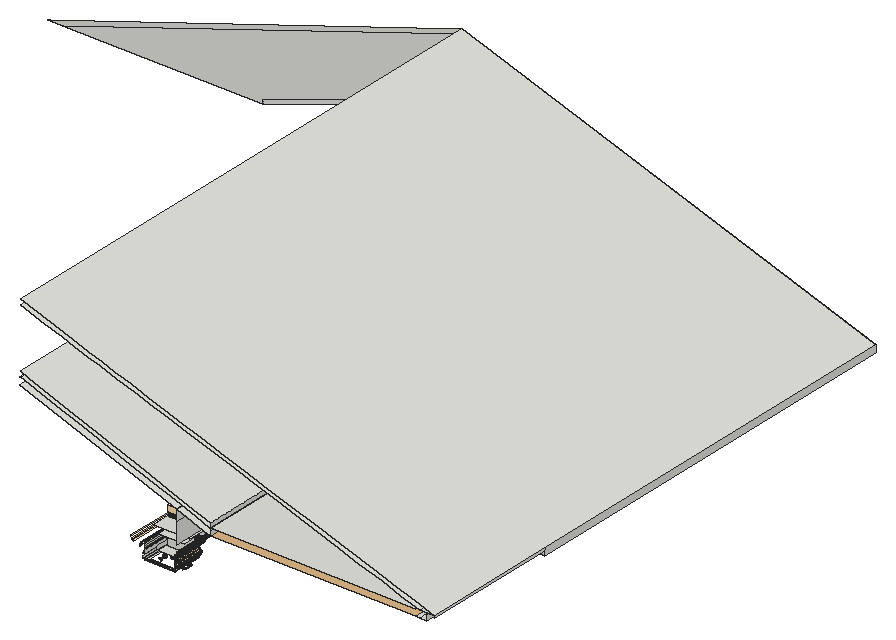
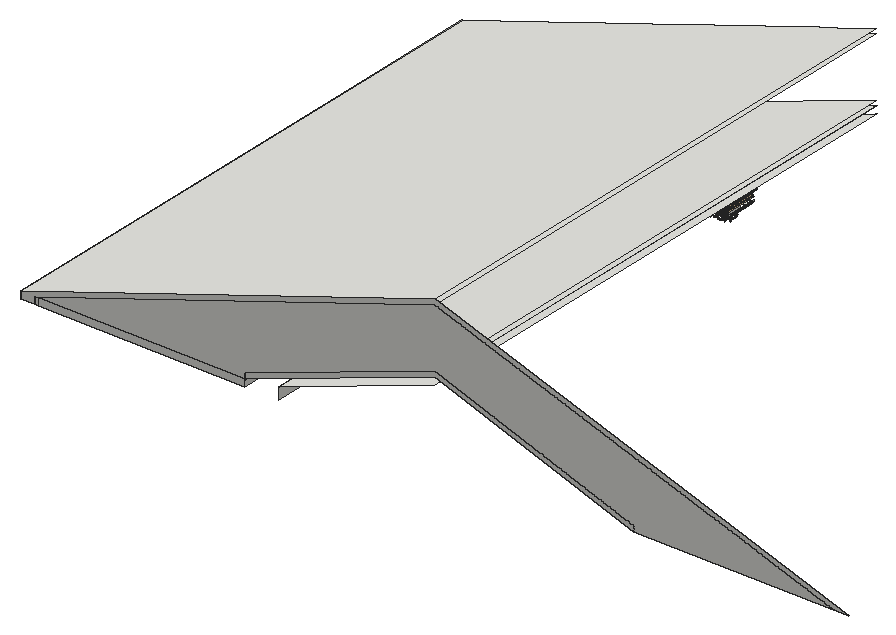
# SketchUp Ruby script. Lengths in inches.
U = 1.inch
M = Sketchup.active_model
def pt(a) = Geom::Point3d.new(a.map { |v| v * U })
def face(e, loops, mat)
  f = e.add_face(loops[0].map { |a| pt(a) })
  loops[1..].each { |l| e.add_face(l.map { |a| pt(a) }).erase! }
  f.material = f.back_material = mat if mat
  f
end
# faces: each face lists its corners as indices into pts; further lists are holes
def faces(e, pts, list, mat = nil) = list.each { |f| face(e, (f[0].is_a?(Array) ? f : [f]).map { |l| l.map { |i| pts[i] } }, mat) }
# xy, xz, yz: faces in a plane at the given z, y or x. An outline is a flat list of corners, or four numbers for a rectangle; further outlines are holes
def ring(l) = l.size == 4 ? [[l[0], l[1]], [l[2], l[1]], [l[2], l[3]], [l[0], l[3]]] : l.each_slice(2).to_a
def flat(e, list, mat, &to3) = list.each { |f| face(e, (f[0].is_a?(Array) ? f : [f]).map { |l| ring(l).map { |u, v| to3.(u, v) } }, mat) }
def xy(e, z, list, mat = nil) = flat(e, list, mat) { |x, y| [x, y, z] }
def xz(e, y, list, mat = nil) = flat(e, list, mat) { |x, z| [x, y, z] }
def yz(e, x, list, mat = nil) = flat(e, list, mat) { |y, z| [x, y, z] }
def lines(e, pts, list) = list.each { |a, b| e.add_line(pt(pts[a]), pt(pts[b])) }
# prism: a flat outline (further loops are holes) pulled along v
def prism(e, loops, v, mat = nil)
  f = face(e, loops, mat); d = Geom::Vector3d.new(v.map { |x| x * U })
  f.pushpull(f.normal.samedirection?(d) ? d.length : -d.length)
end
def box(e, o, s, mat = nil) = prism(e, [[o, [o[0] + s[0], o[1], o[2]], [o[0] + s[0], o[1] + s[1], o[2]], [o[0], o[1] + s[1], o[2]]]], [0, 0, s[2]], mat)
def at(x, y, z, deg = 0) = Geom::Transformation.translation(pt([x, y, z])) * Geom::Transformation.rotation(ORIGIN, Z_AXIS, deg.degrees)
def axes(o, x, y, z) = Geom::Transformation.new([*x, 0, *y, 0, *z, 0, *pt(o).to_a, 1])
def part(name) = M.definitions.add(name)
# library, detail: a bought-in or finely detailed component or shape, given as its bounding box
def library(name, o, s) = part(name).tap { |d| box(d.entities, o, s) }
def detail(e, o, s) = box(e.add_group.entities, o, s)
def put(e, d, t, mat = nil) = e.add_instance(d, t).tap { |i| i.material = mat if mat }
def group(e, t, mat = nil) = e.add_group.tap { |g| g.transformation = t; g.material = mat if mat }.entities
root = M.entities
M.materials.add("[0033_NavajoWhite]").color = [255, 222, 173]
M.materials.add("[0036_BurlyWood]").color = [222, 184, 135]
xy(root,94.95,[[[231.46,8.1,244.45,21.09],[232.25,9.67,243.67,19.51]]])
xy(root,95.99,[[231.46,14.59,244.45,21.09]])
xy(root,95.99,[[[230.94,7.58,244.97,21.61],[231.11,7.74,244.81,21.44]]],"[0033_NavajoWhite]")
xy(root,102.72,[[230.28,22.27,230.08,22.47,245.83,22.47,245.64,22.27]])
xy(root,102.72,[[230.08,22.47,229.3,23.25,246.62,23.25,245.83,22.47]],"[0033_NavajoWhite]")
xy(root,102.86,[[232.25,14.59,243.67,19.51]])
xy(root,105.42,[[230.08,14.59,245.83,22.47]])
xy(root,117,[[351.91,4.75,353.68,64.75],[353.68,4.75,356.68,64.75]])
xy(root,117,[[261.99,4.75,262.6,64.75],[262.6,4.75,351.91,64.75]],"[0036_BurlyWood]")
xy(root,120,[[262.52,4.75,262.6,244.75],[262.6,4.75,351.91,244.75],[353.68,4.75,360,64.75]])
xz(root,19.51,[[232.25,94.95,243.67,102.86]])
xz(root,21.09,[[231.46,94.95,244.45,95.1],[231.46,95.1,244.45,95.99],[231.46,95.99,244.45,97.5625],[231.46,97.5625,244.45,99.87],[231.46,99.87,244.45,100.56],
  [231.46,100.56,244.45,101.46]])
xz(root,21.61,[[230.94,95.99,244.97,96.66]])
xz(root,22.47,[[230.08,102.72,245.83,105.42]])
xz(root,24.44,[[228.12,105.42,247.8,108.125]],"[0033_NavajoWhite]")
xz(root,64.75,[[247.8,117,261.99,117,247.8,122.125],[353.68,117,356.68,120],[356.68,117,360,120]])
xz(root,244.75,[[353.68,117,353.68,120,180,177.89,6.32,120,0,120,180,180,360,120,360,117],[351.91,117,351.91,120,262.6,120,262.6,122.1,180,151.93,93.16,122.1,93.16,120,6.32,120,180,177.89,353.68,120,353.68,117],[262.6,117,351.91,120],[93.16,120,93.16,122.1,180,151.93,262.6,122.1,262.6,120,262.52,120,180,149.8,179.96,149.82]])
yz(root,230.94,[[7.58,95.99,21.61,96.66]])
yz(root,231.46,[[8.1,94.95,21.09,95.1],[8.1,95.1,21.09,95.99],[14.59,95.99,21.09,97.5625],[8.1,97.5625,21.09,99.87],[8.1,99.87,21.09,100.56],
  [8.1,100.56,21.09,101.46]])
yz(root,244.45,[[8.1,94.95,21.09,95.1],[8.1,95.1,21.09,95.99],[14.59,95.99,21.09,97.5625],[8.1,97.5625,21.09,99.87],[8.1,99.87,21.09,100.56],
  [8.1,100.56,21.09,101.46]])
yz(root,244.97,[[7.58,95.99,21.61,96.66]])
yz(root,245.24,[[7.32,96.99,21.87,96.99,21.875,97.11,7.31,97.11],[7.31,97.11,21.875,97.11,21.87,97.23,7.32,97.23]],"[0033_NavajoWhite]")
yz(root,245.83,[[6.73,100.89,22.46,100.89,22.47,101.01,6.72,101.01],[6.72,101.01,22.47,101.01,22.46,101.125,6.73,101.125]],"[0033_NavajoWhite]")
yz(root,247.8,[[4.75,108.125,64.75,117],[4.75,117,64.75,122.125],[64.75,117,244.75,122.125]])
yz(root,262.6,[[4.75,117,244.75,119],[4.75,119,244.75,119.97],[4.75,119.97,244.75,120],[4.75,120,244.75,122.1]])
yz(root,353.68,[[64.75,117,244.75,120]])
yz(root,356.68,[[4.75,117,64.75,119]])
yz(root,360,[[64.75,117,244.75,120],[4.75,119,64.75,120]])
p = [[235.01,18.5625,92.48],[235.01,18.53,92.25],[234.75,18.5625,92.25],[234.76,18.6,92.48],[235.25,18.6,92.48],[235.26,18.5625,92.25],
  [237.96,18.5625,92.48],[237.96,18.53,92.25],[237.7,18.5625,92.25],[237.71,18.6,92.48],[238.2,18.6,92.48],[238.21,18.5625,92.25],
  [240.91,18.5625,92.48],[240.91,18.53,92.25],[240.66,18.5625,92.25],[240.67,18.6,92.48],[241.16,18.6,92.48],[241.17,18.5625,92.25],
  [234.51,18.66,92.25],[234.53,18.69,92.48],[235.48,18.69,92.48],[235.5,18.66,92.25],[237.47,18.66,92.25],[237.48,18.69,92.48],
  [238.43,18.69,92.48],[238.45,18.66,92.25],[240.42,18.66,92.25],[240.4375,18.69,92.48],[241.39,18.69,92.48],[241.4,18.66,92.25],
  [234.31,18.82,92.25],[234.33,18.84,92.48],[235.68,18.84,92.48],[235.7,18.82,92.25],[237.26,18.82,92.25],[237.29,18.84,92.48],
  [238.63,18.84,92.48],[238.65,18.82,92.25],[240.22,18.82,92.25],[240.24,18.84,92.48],[241.58,18.84,92.48],[241.61,18.82,92.25],
  [234.15,19.02,92.25],[234.18,19.04,92.48],[235.83,19.04,92.48],[235.86,19.02,92.25],[237.11,19.02,92.25],[237.14,19.04,92.48],
  [238.78,19.04,92.48],[238.8125,19.02,92.25],[240.06,19.02,92.25],[240.09,19.04,92.48],[241.73,19.04,92.48],[241.76,19.02,92.25],
  [234.05,19.26,92.25],[234.09,19.27,92.48],[235.92,19.27,92.48],[235.96,19.26,92.25],[237.01,19.26,92.25],[237.04,19.27,92.48],
  [238.875,19.27,92.48],[238.91,19.26,92.25],[239.96,19.26,92.25],[239.99,19.27,92.48],[241.83,19.27,92.48],[241.86,19.26,92.25],
  [234.02,19.51,92.25],[234.05,19.51,92.48],[235.96,19.51,92.48],[235.99,19.51,92.25],[236.97,19.51,92.25],[237.01,19.51,92.48],
  [238.91,19.51,92.48],[238.94,19.51,92.25],[239.93,19.51,92.25],[239.96,19.51,92.48],[241.86,19.51,92.48],[241.9,19.51,92.25],
  [233.17,14.84,92.74],[233.2,14.85,92.51],[233.23,14.59,92.51],[233.2,14.59,92.74],[242.72,14.85,92.51],[242.75,14.84,92.74],
  [242.72,14.59,92.74],[242.68,14.59,92.51],[233.07,15.07,92.74],[233.1,15.08,92.51],[242.81,15.08,92.51],[242.84,15.07,92.74],
  [232.92,15.26,92.74],[232.95,15.29,92.51],[242.97,15.29,92.51],[242.99,15.26,92.74],[232.73,15.42,92.74],[232.74,15.44,92.51],
  [243.17,15.44,92.51],[243.19,15.42,92.74],[232.5,15.51,92.74],[232.5,15.54,92.51],[243.41,15.54,92.51],[243.42,15.51,92.74],
  [232.25,15.54,92.74],[232.25,15.58,92.51],[243.67,15.54,92.74],[243.67,15.58,92.51],[232.25,16.59,92.74],[232.5,16.625,92.74],
  [232.5,16.59,92.51],[232.25,16.5625,92.51],[232.73,16.72,92.74],[232.74,16.69,92.51],[243.42,16.625,92.74],[243.41,16.59,92.51],
  [243.17,16.69,92.51],[243.19,16.72,92.74],[243.67,16.59,92.74],[243.67,16.5625,92.51],[232.92,16.875,92.74],[232.95,16.85,92.51],
  [242.97,16.85,92.51],[242.99,16.875,92.74],[233.07,17.07,92.74],[233.1,17.05,92.51],[242.81,17.05,92.51],[242.84,17.07,92.74],
  [233.17,17.3,92.74],[233.2,17.29,92.51],[242.72,17.29,92.51],[242.75,17.3,92.74],[233.2,17.55,92.74],[233.23,17.55,92.51],
  [242.68,17.55,92.51],[242.72,17.55,92.74],[233.17,17.79,92.74],[233.2,17.8,92.51],[242.72,17.8,92.51],[242.75,17.79,92.74],
  [233.07,18.02,92.74],[233.1,18.04,92.51],[242.81,18.04,92.51],[242.84,18.02,92.74],[232.92,18.22,92.74],[232.95,18.24,92.51],
  [242.97,18.24,92.51],[242.99,18.22,92.74],[232.73,18.37,92.74],[232.74,18.4,92.51],[243.17,18.4,92.51],[243.19,18.37,92.74],
  [232.5,18.46,92.74],[232.5,18.5,92.51],[243.41,18.5,92.51],[243.42,18.46,92.74],[232.25,18.53,92.51],[232.25,18.5,92.74],
  [243.67,18.53,92.51],[243.67,18.5,92.74],[234.78,18.69,92.7],[234.58,18.78,92.7],[235.01,18.66,92.7],[235.23,18.69,92.7],
  [235.43,18.78,92.7],[237.74,18.69,92.7],[237.53,18.78,92.7],[237.96,18.66,92.7],[238.18,18.69,92.7],[238.38,18.78,92.7],
  [240.69,18.69,92.7],[240.48,18.78,92.7],[240.91,18.66,92.7],[241.13,18.69,92.7],[241.34,18.78,92.7],[234.4,18.91,92.7],
  [235.61,18.91,92.7],[237.36,18.91,92.7],[238.5625,18.91,92.7],[240.31,18.91,92.7],[241.51,18.91,92.7],[234.27,19.09,92.7],
  [235.74,19.09,92.7],[237.22,19.09,92.7],[238.7,19.09,92.7],[240.17,19.09,92.7],[241.65,19.09,92.7],[234.18,19.29,92.7],
  [235.83,19.29,92.7],[237.14,19.29,92.7],[238.78,19.29,92.7],[240.09,19.29,92.7],[241.73,19.29,92.7],[234.15,19.51,92.7],
  [235.86,19.51,92.7],[237.11,19.51,92.7],[238.8125,19.51,92.7],[240.06,19.51,92.7],[241.76,19.51,92.7],[233.07,14.8125,92.96],
  [233.1,14.59,92.96],[242.84,14.8125,92.96],[242.81,14.59,92.96],[232.99,15.02,92.96],[242.93,15.02,92.96],[232.85,15.2,92.96],
  [243.0625,15.2,92.96],[232.68,15.33,92.96],[243.24,15.33,92.96],[232.47,15.42,92.96],[243.45,15.42,92.96],[232.25,15.44,92.96],
  [243.67,15.44,92.96],[232.25,16.69,92.96],[232.47,16.72,92.96],[232.68,16.81,92.96],[243.45,16.72,92.96],[243.24,16.81,92.96],
  [243.67,16.69,92.96],[232.85,16.94,92.96],[243.0625,16.94,92.96],[232.99,17.12,92.96],[242.93,17.12,92.96],[233.07,17.32,92.96],
  [242.84,17.32,92.96],[233.1,17.55,92.96],[242.81,17.55,92.96],[233.07,17.77,92.96],[242.84,17.77,92.96],[232.99,17.97,92.96],
  [242.93,17.97,92.96],[232.85,18.15,92.96],[243.0625,18.15,92.96],[232.68,18.28,92.96],[243.24,18.28,92.96],[232.47,18.37,92.96],
  [243.45,18.37,92.96],[232.25,18.4,92.96],[243.67,18.4,92.96],[234.83,18.84,92.89],[234.66,18.91,92.89],[235.01,18.82,92.89],
  [235.1875,18.84,92.89],[235.35,18.91,92.89],[237.78,18.84,92.89],[237.61,18.91,92.89],[237.96,18.82,92.89],[238.14,18.84,92.89],
  [238.31,18.91,92.89],[240.73,18.84,92.89],[240.5625,18.91,92.89],[240.91,18.82,92.89],[241.09,18.84,92.89],[241.26,18.91,92.89],
  [234.51,19.02,92.89],[235.5,19.02,92.89],[237.47,19.02,92.89],[238.45,19.02,92.89],[240.42,19.02,92.89],[241.4,19.02,92.89],
  [234.4,19.17,92.89],[235.61,19.17,92.89],[237.36,19.17,92.89],[238.5625,19.17,92.89],[240.31,19.17,92.89],[241.51,19.17,92.89],
  [234.33,19.33,92.89],[235.68,19.33,92.89],[237.29,19.33,92.89],[238.63,19.33,92.89],[240.24,19.33,92.89],[241.58,19.33,92.89],
  [234.31,19.51,92.89],[235.7,19.51,92.89],[237.26,19.51,92.89],[238.65,19.51,92.89],[240.22,19.51,92.89],[241.61,19.51,92.89],
  [234.88,19.04,93.03],[234.76,19.09,93.03],[235.01,19.02,93.03],[235.13,19.04,93.03],[235.25,19.09,93.03],[237.83,19.04,93.03],
  [237.71,19.09,93.03],[237.96,19.02,93.03],[238.09,19.04,93.03],[238.2,19.09,93.03],[240.78,19.04,93.03],[240.67,19.09,93.03],
  [240.91,19.02,93.03],[241.04,19.04,93.03],[241.16,19.09,93.03],[234.66,19.17,93.03],[235.35,19.17,93.03],[237.61,19.17,93.03],
  [238.31,19.17,93.03],[240.5625,19.17,93.03],[241.26,19.17,93.03],[234.58,19.27,93.03],[235.43,19.27,93.03],[237.53,19.27,93.03],
  [238.38,19.27,93.03],[240.48,19.27,93.03],[241.34,19.27,93.03],[234.53,19.39,93.03],[235.48,19.39,93.03],[237.48,19.39,93.03],
  [238.43,19.39,93.03],[240.4375,19.39,93.03],[241.39,19.39,93.03],[234.51,19.51,93.03],[235.5,19.51,93.03],[237.47,19.51,93.03],
  [238.45,19.51,93.03],[240.42,19.51,93.03],[241.4,19.51,93.03],[232.92,14.77,93.15],[232.95,14.59,93.15],[242.99,14.77,93.15],
  [242.97,14.59,93.15],[232.85,14.94,93.15],[243.0625,14.94,93.15],[232.74,15.08,93.15],[243.17,15.08,93.15],[232.6,15.2,93.15],
  [243.32,15.2,93.15],[232.43,15.26,93.15],[243.49,15.26,93.15],[232.25,15.29,93.15],[243.67,15.29,93.15],[232.25,16.85,93.15],
  [232.43,16.875,93.15],[232.6,16.94,93.15],[243.49,16.875,93.15],[243.32,16.94,93.15],[243.67,16.85,93.15],[232.74,17.05,93.15],
  [243.17,17.05,93.15],[232.85,17.2,93.15],[243.0625,17.2,93.15],[232.92,17.37,93.15],[242.99,17.37,93.15],[232.95,17.55,93.15],
  [242.97,17.55,93.15],[232.92,17.73,93.15],[242.99,17.73,93.15],[232.85,17.89,93.15],[243.0625,17.89,93.15],[232.74,18.04,93.15],
  [243.17,18.04,93.15],[232.6,18.15,93.15],[243.32,18.15,93.15],[232.43,18.22,93.15],[243.49,18.22,93.15],[232.25,18.24,93.15],
  [243.67,18.24,93.15],[234.94,19.27,93.12],[234.88,19.29,93.12],[235.01,19.26,93.12],[235.07,19.27,93.12],[235.13,19.29,93.12],
  [237.89,19.27,93.12],[237.83,19.29,93.12],[237.96,19.26,93.12],[238.02,19.27,93.12],[238.09,19.29,93.12],[240.85,19.27,93.12],
  [240.78,19.29,93.12],[240.91,19.26,93.12],[240.98,19.27,93.12],[241.04,19.29,93.12],[234.83,19.33,93.12],[235.1875,19.33,93.12],
  [237.78,19.33,93.12],[238.14,19.33,93.12],[240.73,19.33,93.12],[241.09,19.33,93.12],[234.78,19.39,93.12],[235.23,19.39,93.12],
  [237.74,19.39,93.12],[238.18,19.39,93.12],[240.69,19.39,93.12],[241.13,19.39,93.12],[234.76,19.45,93.12],[235.25,19.45,93.12],
  [237.71,19.45,93.12],[238.2,19.45,93.12],[240.67,19.45,93.12],[241.16,19.45,93.12],[234.75,19.51,93.12],[235.26,19.51,93.12],
  [237.7,19.51,93.12],[238.21,19.51,93.12],[240.66,19.51,93.12],[241.17,19.51,93.12],[232.73,14.72,93.29],[232.74,14.59,93.29],
  [243.19,14.72,93.29],[243.17,14.59,93.29],[232.68,14.84,93.29],[243.24,14.84,93.29],[232.6,14.94,93.29],[243.32,14.94,93.29],
  [232.5,15.02,93.29],[243.42,15.02,93.29],[232.38,15.07,93.29],[243.54,15.07,93.29],[232.25,15.08,93.29],[243.67,15.08,93.29],
  [232.25,17.05,93.29],[232.38,17.07,93.29],[243.54,17.07,93.29],[243.67,17.05,93.29],[232.5,17.12,93.29],[232.6,17.2,93.29],
  [243.42,17.12,93.29],[243.32,17.2,93.29],[232.68,17.3,93.29],[243.24,17.3,93.29],[232.73,17.42,93.29],[243.19,17.42,93.29],
  [232.74,17.55,93.29],[243.17,17.55,93.29],[232.73,17.67,93.29],[243.19,17.67,93.29],[232.68,17.79,93.29],[243.24,17.79,93.29],
  [232.6,17.89,93.29],[243.32,17.89,93.29],[232.5,17.97,93.29],[243.42,17.97,93.29],[232.38,18.02,93.29],[232.25,18.04,93.29],
  [243.54,18.02,93.29],[243.67,18.04,93.29],[235.01,19.51,93.15],[237.96,19.51,93.15],[240.91,19.51,93.15],[232.5,14.66,93.38],
  [232.5,14.59,93.38],[243.42,14.66,93.38],[243.41,14.59,93.38],[232.43,14.77,93.38],[232.47,14.72,93.38],[243.45,14.72,93.38],
  [243.49,14.77,93.38],[232.32,14.84,93.38],[232.25,14.85,93.38],[232.38,14.8125,93.38],[243.54,14.8125,93.38],[243.6,14.84,93.38],
  [243.67,14.85,93.38],[232.25,17.29,93.38],[232.32,17.3,93.38],[232.38,17.32,93.38],[232.43,17.37,93.38],[243.54,17.32,93.38],
  [243.49,17.37,93.38],[243.6,17.3,93.38],[243.67,17.29,93.38],[232.47,17.42,93.38],[243.45,17.42,93.38],[232.5,17.48,93.38],
  [243.42,17.48,93.38],[232.5,17.55,93.38],[243.41,17.55,93.38],[232.5,17.61,93.38],[243.42,17.61,93.38],[232.47,17.67,93.38],
  [243.45,17.67,93.38],[232.43,17.73,93.38],[232.38,17.77,93.38],[243.49,17.73,93.38],[243.54,17.77,93.38],[232.32,17.79,93.38],
  [232.25,17.8,93.38],[243.6,17.79,93.38],[243.67,17.8,93.38],[232.25,14.59,93.41],[243.67,14.59,93.41],[232.25,17.55,93.41],
  [243.67,17.55,93.41],[231.45,8.09,95.25],[231.45,21.1,95.25],[231.46,21.09,95.1],[231.46,8.1,95.1],[244.45,8.1,95.1],
  [244.45,21.09,95.1],[244.47,21.1,95.25],[244.47,8.09,95.25],[231.43,8.06,95.4],[231.43,21.12,95.4],[244.49,21.12,95.4],
  [244.49,8.06,95.4],[244.52,21.15,95.53],[231.4,21.15,95.53],[244.55,21.1875,95.66],[231.36,21.1875,95.66],[244.6,21.24,95.77],
  [231.32,21.24,95.77],[231.26,7.9,95.86],[231.26,21.29,95.86],[231.32,7.95,95.77],[244.6,7.95,95.77],[244.65,21.29,95.86],
  [244.65,7.9,95.86],[231.2,7.84,95.93],[231.2,21.35,95.93],[244.71,21.35,95.93],[244.71,7.84,95.93],[244.78,21.41,95.98],
  [231.14,21.41,95.98],[231.11,7.74,95.99],[231.11,21.44,95.99],[231.14,7.78,95.98],[244.78,7.78,95.98],[244.81,21.44,95.99],
  [244.81,7.74,95.99],[245.1,7.45,96.68],[245.1,21.73,96.68],[245.14,21.78,96.72],[245.14,7.41,96.72],[245.04,7.51,96.66],
  [245.04,21.68,96.66],[230.87,21.68,96.66],[230.82,21.73,96.68],[230.77,21.78,96.72],[245.18,21.82,96.79],[230.73,21.82,96.79],
  [245.22,21.85,96.89],[230.7,21.85,96.89],[245.22,7.34,96.89],[245.24,21.87,96.99],[245.24,7.32,96.99],[230.68,21.87,96.99],
  [245.24,21.875,97.11],[230.67,21.875,97.11],[245.24,21.87,97.23],[230.68,21.87,97.23],[245.24,7.32,97.23],[245.22,21.85,97.34],
  [245.22,7.34,97.34],[230.7,21.85,97.34],[245.18,21.82,97.43],[230.73,21.82,97.43],[245.14,21.78,97.5],[230.77,21.78,97.5],
  [245.14,7.41,97.5],[245.1,21.73,97.55],[245.1,7.45,97.55],[245.04,21.68,97.5625],[245.04,7.51,97.5625],[230.82,21.73,97.55],
  [230.87,21.68,97.5625],[244.95,21.58,97.74],[244.95,7.61,97.74],[230.97,21.58,97.74],[231.0625,7.7,97.93],[231.0625,21.49,97.93],
  [230.97,7.61,97.74],[244.85,21.49,97.93],[244.85,7.7,97.93],[244.77,21.4,98.14],[244.77,7.78,98.14],[231.15,21.4,98.14],
  [231.22,7.86,98.375],[231.22,21.33,98.375],[231.15,7.78,98.14],[244.69,21.33,98.375],[244.69,7.86,98.375],[231.29,7.92,98.62],
  [231.29,21.26,98.62],[244.625,21.26,98.62],[244.625,7.92,98.62],[231.35,7.98,98.875],[231.35,21.2,98.875],[244.57,21.2,98.875],
  [244.57,7.98,98.875],[231.39,8.03,99.14],[231.39,21.16,99.14],[244.52,21.16,99.14],[244.52,8.03,99.14],[231.43,8.0625,99.42],
  [231.43,21.12,99.42],[244.49,21.12,99.42],[244.49,8.0625,99.42],[244.46,21.1,99.7],[231.45,21.1,99.7],[231.46,8.1,99.87],
  [231.46,21.09,99.87],[231.45,8.09,99.7],[244.46,8.09,99.7],[244.45,21.09,99.87],[244.45,8.1,99.87],[230.14,6.78,100.6875],
  [230.14,22.41,100.6875],[230.18,22.37,100.62],[230.18,6.82,100.62],[230.23,22.32,100.57],[230.23,6.86,100.57],[245.6875,6.86,100.57],
  [245.6875,22.32,100.57],[245.73,22.37,100.62],[245.73,6.82,100.62],[245.77,22.41,100.6875],[245.77,6.78,100.6875],[245.64,6.92,100.56],
  [245.64,22.27,100.56],[230.28,22.27,100.56],[245.81,22.44,100.78],[245.81,6.74,100.78],[230.11,22.44,100.78],[245.83,22.46,100.89],
  [230.09,22.46,100.89],[245.83,22.47,101.01],[230.08,22.47,101.01],[245.83,22.46,101.125],[230.09,22.46,101.125],[245.81,22.44,101.23],
  [230.11,22.44,101.23],[245.81,6.74,101.23],[245.77,22.41,101.33],[245.77,6.78,101.33],[230.14,22.41,101.33],[230.18,6.82,101.4],
  [230.18,22.37,101.4],[230.14,6.78,101.33],[245.73,22.37,101.4],[245.73,6.82,101.4],[230.23,6.86,101.44],[230.23,22.32,101.44],
  [245.6875,22.32,101.44],[245.6875,6.86,101.44],[245.64,22.27,101.46],[245.64,6.92,101.46],[230.28,22.27,101.46],[245.53,22.17,101.6],
  [245.53,7.02,101.6],[245.58,6.97,101.52],[245.58,22.22,101.52],[230.34,22.22,101.52],[230.38,22.17,101.6],[245.49,22.13,101.7],
  [245.49,7.06,101.7],[230.42,22.13,101.7],[245.46,22.1,101.82],[245.46,7.09,101.82],[230.45,22.1,101.82],[230.45,7.09,101.82],
  [230.47,7.11,101.95],[230.47,22.08,101.95],[245.44,22.08,101.95],[245.44,7.11,101.95],[230.48,7.11,102.09],[230.48,22.07,102.09],
  [245.4375,22.07,102.09],[245.4375,7.11,102.09],[230.47,7.11,102.23],[230.47,22.08,102.23],[245.44,22.08,102.23],[245.44,7.11,102.23],
  [230.45,7.09,102.36],[230.45,22.1,102.36],[245.46,22.1,102.36],[245.46,7.09,102.36],[245.49,22.13,102.48],[245.49,7.06,102.48],
  [230.42,22.13,102.48],[245.53,22.17,102.58],[245.53,7.02,102.58],[230.38,22.17,102.58],[245.58,22.22,102.66],[245.58,6.97,102.66],
  [230.34,22.22,102.66],[246.78,5.77,102.7],[246.78,23.41,102.7],[246.94,23.58,102.73],[246.94,5.61,102.73],[246.62,5.93,102.72],
  [246.62,23.25,102.72],[230.28,22.27,102.72],[245.64,22.27,102.72],[229.3,23.25,102.72],[229.14,23.41,102.7],[228.98,23.58,102.73],
  [228.82,23.73,102.82],[247.1,23.73,102.82],[247.1,5.45,102.82],[247.25,23.88,102.96],[247.25,5.3,102.96],[228.67,23.88,102.96],
  [228.53,5.17,103.15],[228.53,24.02,103.15],[228.67,5.3,102.96],[247.38,24.02,103.15],[247.38,5.17,103.15],[247.51,24.14,103.39],
  [247.51,5.05,103.39],[228.41,24.14,103.39],[247.61,24.24,103.68],[247.61,4.94,103.68],[228.31,24.24,103.68],[228.22,4.86,103.99],
  [228.22,24.33,103.99],[228.31,4.94,103.68],[247.7,24.33,103.99],[247.7,4.86,103.99],[247.76,24.39,104.33],[247.76,4.79,104.33],
  [228.16,24.39,104.33],[247.8,24.43,104.6875],[247.8,4.75,104.6875],[228.12,24.43,104.6875],[228.11,4.74,105.05],[228.11,24.45,105.05],
  [228.12,4.75,104.6875],[247.8125,24.45,105.05],[247.8125,4.74,105.05],[247.8,24.44,105.42],[247.8,4.75,105.42],[228.12,24.44,105.42],
  [261.99,4.75,117],[247.8,4.75,122.125],[247.8,64.75,122.125],[261.99,64.75,117],[180,4.75,177.89],[190.82,4.75,174.29],
  [198.59,4.75,171.69],[203.74,4.75,169.98],[209.51,4.75,168.05],[214.75,4.75,166.31],[222.01,4.75,163.89],[229.64,4.75,161.35],
  [236.39,4.75,159.09],[244.33,4.75,156.45],[252.34,4.75,153.78],[262.54,4.75,150.38],[271.37,4.75,147.4375],[281.28,4.75,144.13],
  [291.76,4.75,140.64],[303.43,4.75,136.75],[316.44,4.75,132.41],[327.22,4.75,128.82],[337.3,4.75,125.46],[345.49,4.75,122.73],
  [353.68,4.75,120],[353.68,64.75,120],[353.68,244.75,120],[180,244.75,177.89],[351.8125,4.75,122.73],[360,4.75,120],
  [360,64.75,120],[360,244.75,120],[180,244.75,180],[180,4.75,180],[197,4.75,174.33],[204.77,4.75,171.74],
  [209.93,4.75,170.02],[215.69,4.75,168.1],[221.07,4.75,166.31],[228.33,4.75,163.89],[235.96,4.75,161.35],[242.72,4.75,159.09],
  [250.66,4.75,156.45],[258.67,4.75,153.78],[268.86,4.75,150.38],[277.69,4.75,147.4375],[287.61,4.75,144.13],[298.08,4.75,140.64],
  [309.76,4.75,136.75],[322.77,4.75,132.41],[333.54,4.75,128.82],[343.625,4.75,125.46],[180,244.75,149.8],[180,4.75,149.8],
  [186.55,4.75,147.4375],[195.7,4.75,144.13],[205.37,4.75,140.64],[216.15,4.75,136.75],[228.15,4.75,132.41],[238.1,4.75,128.82],
  [247.4,4.75,125.46],[256.71,4.75,122.1],[262.52,4.75,120],[262.52,244.75,120],[262.6,4.75,119.97],[262.6,244.75,119.97],
  [184.29,4.75,150.38],[180,4.75,151.93],[180,244.75,151.93],[262.6,244.75,122.1],[262.6,4.75,122.1],[253.29,4.75,125.46],
  [243.99,4.75,128.82],[234.04,4.75,132.41],[222.03,4.75,136.75],[211.26,4.75,140.64],[201.59,4.75,144.13],[192.4375,4.75,147.4375],
  [179.96,244.75,146.625],[179.96,4.75,146.625],[247.8,244.75,122.125],[179.96,4.75,149.82],[179.96,244.75,149.82],[351.91,64.75,117],
  [351.91,244.75,117],[244.84,14.59,96.01],[244.91,14.59,96.01]]
faces(root,p,[[0,1,2,3],[4,5,1,0],[6,7,8,9],[10,11,7,6],[12,13,14,15],[16,17,13,12],[3,2,18,19],[20,21,5,4],
  [9,8,22,23],[24,25,11,10],[15,14,26,27],[28,29,17,16],[19,18,30,31],[32,33,21,20],[23,22,34,35],[36,37,25,24],
  [27,26,38,39],[40,41,29,28],[31,30,42,43],[44,45,33,32],[35,34,46,47],[48,49,37,36],[39,38,50,51],[52,53,41,40],
  [43,42,54,55],[56,57,45,44],[47,46,58,59],[60,61,49,48],[51,50,62,63],[64,65,53,52],[54,66,67,55],[56,68,69,57],
  [58,70,71,59],[60,72,73,61],[62,74,75,63],[64,76,77,65],[78,79,80,81],[82,83,84,85],[86,87,79,78],[88,89,83,82],
  [90,91,87,86],[92,93,89,88],[94,95,91,90],[96,97,93,92],[98,99,95,94],[100,101,97,96],[98,102,103,99],[104,101,100,105],
  [106,107,108,109],[108,107,110,111],[112,113,114,115],[112,116,117,113],[111,110,118,119],[115,114,120,121],[119,118,122,123],[121,120,124,125],
  [123,122,126,127],[125,124,128,129],[127,126,130,131],[129,128,132,133],[131,130,134,135],[133,132,136,137],[135,134,138,139],[137,136,140,141],
  [139,138,142,143],[141,140,144,145],[143,142,146,147],[145,144,148,149],[147,146,150,151],[149,148,152,153],[154,151,150,155],[152,156,157,153],
  [158,3,19,159],[160,0,3,158],[161,4,0,160],[162,20,4,161],[163,9,23,164],[165,6,9,163],[166,10,6,165],[167,24,10,166],
  [168,15,27,169],[170,12,15,168],[171,16,12,170],[172,28,16,171],[159,19,31,173],[174,32,20,162],[164,23,35,175],[176,36,24,167],
  [169,27,39,177],[178,40,28,172],[173,31,43,179],[180,44,32,174],[175,35,47,181],[182,48,36,176],[177,39,51,183],[184,52,40,178],
  [179,43,55,185],[186,56,44,180],[181,47,59,187],[188,60,48,182],[183,51,63,189],[190,64,52,184],[55,67,191,185],[186,192,68,56],
  [59,71,193,187],[188,194,72,60],[63,75,195,189],[190,196,76,64],[197,78,81,198],[83,199,200,84],[201,86,78,197],[89,202,199,83],
  [203,90,86,201],[93,204,202,89],[205,94,90,203],[97,206,204,93],[207,98,94,205],[101,208,206,97],[207,209,102,98],[210,208,101,104],
  [211,212,107,106],[107,212,213,110],[214,112,115,215],[214,216,116,112],[110,213,217,118],[215,115,121,218],[118,217,219,122],[218,121,125,220],
  [122,219,221,126],[220,125,129,222],[126,221,223,130],[222,129,133,224],[130,223,225,134],[224,133,137,226],[134,225,227,138],[226,137,141,228],
  [138,227,229,142],[228,141,145,230],[142,229,231,146],[230,145,149,232],[146,231,233,150],[232,149,153,234],[155,150,233,235],[153,157,236,234],
  [237,158,159,238],[239,160,158,237],[240,161,160,239],[241,162,161,240],[242,163,164,243],[244,165,163,242],[245,166,165,244],[246,167,166,245],
  [247,168,169,248],[249,170,168,247],[250,171,170,249],[251,172,171,250],[238,159,173,252],[253,174,162,241],[243,164,175,254],[255,176,167,246],
  [248,169,177,256],[257,178,172,251],[252,173,179,258],[259,180,174,253],[254,175,181,260],[261,182,176,255],[256,177,183,262],[263,184,178,257],
  [258,179,185,264],[265,186,180,259],[260,181,187,266],[267,188,182,261],[262,183,189,268],[269,190,184,263],[185,191,270,264],[265,271,192,186],
  [187,193,272,266],[267,273,194,188],[189,195,274,268],[269,275,196,190],[276,237,238,277],[278,239,237,276],[279,240,239,278],[280,241,240,279],
  [281,242,243,282],[283,244,242,281],[284,245,244,283],[285,246,245,284],[286,247,248,287],[288,249,247,286],[289,250,249,288],[290,251,250,289],
  [277,238,252,291],[292,253,241,280],[282,243,254,293],[294,255,246,285],[287,248,256,295],[296,257,251,290],[291,252,258,297],[298,259,253,292],
  [293,254,260,299],[300,261,255,294],[295,256,262,301],[302,263,257,296],[297,258,264,303],[304,265,259,298],[299,260,266,305],[306,267,261,300],
  [301,262,268,307],[308,269,263,302],[264,270,309,303],[304,310,271,265],[266,272,311,305],[306,312,273,267],[268,274,313,307],[308,314,275,269],
  [315,197,198,316],[199,317,318,200],[319,201,197,315],[202,320,317,199],[321,203,201,319],[204,322,320,202],[323,205,203,321],[206,324,322,204],
  [325,207,205,323],[208,326,324,206],[325,327,209,207],[328,326,208,210],[329,330,212,211],[212,330,331,213],[332,214,215,333],[332,334,216,214],
  [213,331,335,217],[333,215,218,336],[217,335,337,219],[336,218,220,338],[219,337,339,221],[338,220,222,340],[221,339,341,223],[340,222,224,342],
  [223,341,343,225],[342,224,226,344],[225,343,345,227],[344,226,228,346],[227,345,347,229],[346,228,230,348],[229,347,349,231],[348,230,232,350],
  [231,349,351,233],[350,232,234,352],[235,233,351,353],[234,236,354,352],[355,276,277,356],[357,278,276,355],[358,279,278,357],[359,280,279,358],
  [360,281,282,361],[362,283,281,360],[363,284,283,362],[364,285,284,363],[365,286,287,366],[367,288,286,365],[368,289,288,367],[369,290,289,368],
  [356,277,291,370],[371,292,280,359],[361,282,293,372],[373,294,285,364],[366,287,295,374],[375,296,290,369],[370,291,297,376],[377,298,292,371],
  [372,293,299,378],[379,300,294,373],[374,295,301,380],[381,302,296,375],[376,297,303,382],[383,304,298,377],[378,299,305,384],[385,306,300,379],
  [380,301,307,386],[387,308,302,381],[303,309,388,382],[383,389,310,304],[305,311,390,384],[385,391,312,306],[307,313,392,386],[387,393,314,308],
  [394,315,316,395],[317,396,397,318],[398,319,315,394],[320,399,396,317],[400,321,319,398],[322,401,399,320],[402,323,321,400],[324,403,401,322],
  [404,325,323,402],[326,405,403,324],[404,406,327,325],[407,405,326,328],[408,409,330,329],[410,411,334,332],[330,409,412,331],[331,412,413,335],
  [414,333,336,415],[410,332,333,414],[335,413,416,337],[415,336,338,417],[337,416,418,339],[417,338,340,419],[339,418,420,341],[419,340,342,421],
  [341,420,422,343],[421,342,344,423],[343,422,424,345],[423,344,346,425],[345,424,426,347],[425,346,348,427],[347,426,428,349],[427,348,350,429],
  [353,351,430,431],[349,428,430,351],[429,350,352,432],[352,354,433,432],[434,356,370],[434,370,376],[434,357,355],[434,355,356],
  [434,358,357],[434,359,358],[434,371,359],[434,377,371],[435,372,378],[435,360,361],[435,361,372],[435,362,360],
  [435,363,362],[435,364,363],[435,373,364],[435,379,373],[436,366,374],[436,374,380],[436,367,365],[436,365,366],
  [436,368,367],[436,369,368],[436,375,369],[436,381,375],[434,376,382],[382,388,434],[434,383,377],[383,434,389],
  [435,378,384],[384,390,435],[435,385,379],[385,435,391],[436,380,386],[386,392,436],[436,387,381],[387,436,393],
  [437,394,395,438],[396,439,440,397],[441,400,398,442],[442,398,394,437],[399,443,439,396],[401,444,443,399],[445,446,406,404],[445,404,402,447],
  [447,402,400,441],[403,448,444,401],[405,449,448,403],[450,449,405,407],[451,452,409,408],[409,452,453,412],[412,453,454,413],[455,414,415,456],
  [457,410,414,455],[457,458,411,410],[413,454,459,416],[456,415,417,460],[416,459,461,418],[460,417,419,462],[418,461,463,420],[462,419,421,464],
  [420,463,465,422],[464,421,423,466],[422,465,467,424],[466,423,425,468],[424,467,469,426],[426,469,470,428],[468,425,427,471],[471,427,429,472],
  [431,430,473,474],[428,470,473,430],[472,429,432,475],[432,433,476,475],[477,437,438],[477,442,437],[477,441,442],[477,447,441],
  [477,445,447],[445,477,446],[439,478,440],[443,478,439],[444,478,443],[448,478,444],[449,478,448],[478,449,450],
  [479,452,451],[452,479,453],[453,479,454],[480,457,455],[480,455,456],[457,480,458],[454,479,459],[459,479,461],
  [480,456,460],[480,460,462],[461,479,463],[463,479,465],[465,479,467],[467,479,469],[469,479,470],[470,479,473],
  [474,473,479],[480,462,464],[480,464,466],[480,466,468],[480,468,471],[480,471,472],[480,472,475],[475,476,480],
  [635,636,637,638],[639,640,635,638],[634,639,638,632],[641,642,636,635],[640,643,641,635],[644,645,642,641],[643,646,644,641],[646,647,648,649],
  [650,651,645,644],[646,649,650,644],[649,648,652,653],[654,655,651,650],[649,653,654,650],[653,652,656,657],[658,659,655,654],[653,657,658,654],
  [657,656,660,661],[662,663,659,658],[657,661,662,658],[664,665,663,662],[661,666,664,662],[667,668,665,664],[666,669,667,664],[670,671,668,667],
  [669,672,670,667],[672,679,680,670],[720,721,722,723],[724,725,726,727,728,729,730,731,732,733,734,735,736,737,738,739,740,741,742,743,744,745,746,747],[748,749,750,751,752,753,754,755,756,757,758,759,760,761,762,763,764,765,766,767,768,769,770,771],[772,773,774,775,776,777,778,779,780,781,782,783],[783,782,784,785],[786,787,788,789,790,791,792,793,794,795,796,797],
  [798,799,721,722,800],[773,801,802,772]])
faces(root,p,[[481,482,483,484],[485,486,487,488],[487,486,483,482],[489,490,482,481],[488,487,491,492],[491,487,482,490],[493,491,490,494],[495,493,494,496],
  [497,495,496,498],[499,500,498,501],[502,497,503,504],[503,497,498,500],[505,506,500,499],[504,503,507,508],[509,507,506,510],[507,503,500,506],
  [511,512,510,513],[514,509,515,516],[515,509,510,512],[517,518,519,520],[521,522,518,517],[518,522,523,524],[519,518,524,525],[526,519,525,527],
  [528,526,527,529],[530,528,531,532],[531,528,529,533],[534,531,533,535],[536,534,535,537],[538,536,539,540],[539,536,537,541],[542,539,541,543],
  [544,542,543,545],[546,544,547,548],[548,547,549,550],[549,547,551,552],[547,544,545,551],[550,549,553,554],[553,549,552,555],[556,557,555,558],
  [554,553,559,560],[559,553,555,557],[560,559,561,562],[561,559,557,563],[564,565,563,566],[562,561,567,568],[567,561,563,565],[569,570,565,564],
  [568,567,571,572],[571,567,565,570],[573,574,570,569],[572,571,575,576],[575,571,570,574],[577,578,574,573],[576,575,579,580],[579,575,574,578],
  [581,582,578,577],[580,579,583,584],[583,579,578,582],[585,583,582,586],[587,588,586,589],[590,585,591,592],[591,585,586,588],[593,594,595,596],
  [596,595,597,598],[599,600,601,602],[602,601,603,604],[605,606,600,599],[600,606,607,597],[601,600,597,595],[603,601,595,594],[604,603,608,609],
  [608,603,594,610],[611,608,610,612],[613,611,612,614],[615,613,614,616],[617,615,616,618],[619,617,620,621],[620,617,618,622],[623,624,622,625],
  [620,626,627,621],[626,620,622,624],[628,629,624,623],[627,626,630,631],[631,630,632,633],[632,630,629,634],[630,626,624,629],[673,674,675,676],
  [677,678,674,673],[681,682,674,678],[682,683,675,674],[683,684,685,675],[686,685,687,688],[684,689,687,685],[690,691,689,692],[688,687,693,694],
  [689,691,693,687],[694,693,695,696],[691,697,695,693],[696,695,698,699],[697,700,698,695],[701,702,700,703],[699,698,704,705],[700,702,704,698],
  [705,704,706,707],[702,708,706,704],[707,706,709,710],[708,711,709,706],[712,713,711,714],[710,709,715,716],[711,713,715,709],[716,715,717,718],
  [713,719,717,715]],"[0033_NavajoWhite]")
lines(root,p,[[803,804],[805,806]])
